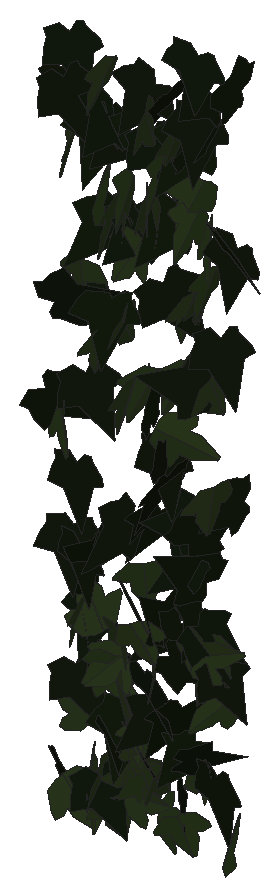
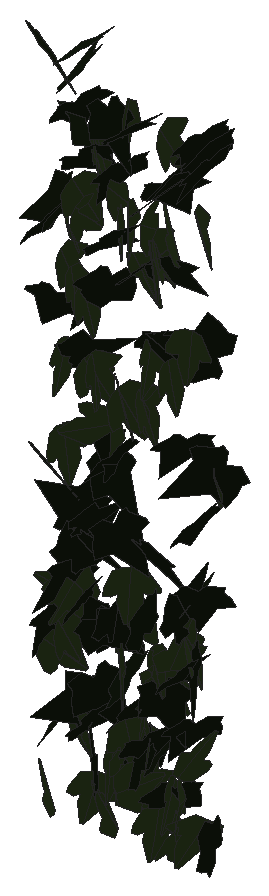
# SketchUp Ruby script. Lengths in inches.
U = 1.inch
M = Sketchup.active_model
def pt(a) = Geom::Point3d.new(a.map { |v| v * U })
def face(e, loops, mat)
  f = e.add_face(loops[0].map { |a| pt(a) })
  loops[1..].each { |l| e.add_face(l.map { |a| pt(a) }).erase! }
  f.material = f.back_material = mat if mat
  f
end
# faces: each face lists its corners as indices into pts; further lists are holes
def faces(e, pts, list, mat = nil) = list.each { |f| face(e, (f[0].is_a?(Array) ? f : [f]).map { |l| l.map { |i| pts[i] } }, mat) }
# xy, xz, yz: faces in a plane at the given z, y or x. An outline is a flat list of corners, or four numbers for a rectangle; further outlines are holes
def ring(l) = l.size == 4 ? [[l[0], l[1]], [l[2], l[1]], [l[2], l[3]], [l[0], l[3]]] : l.each_slice(2).to_a
def flat(e, list, mat, &to3) = list.each { |f| face(e, (f[0].is_a?(Array) ? f : [f]).map { |l| ring(l).map { |u, v| to3.(u, v) } }, mat) }
def xy(e, z, list, mat = nil) = flat(e, list, mat) { |x, y| [x, y, z] }
def xz(e, y, list, mat = nil) = flat(e, list, mat) { |x, z| [x, y, z] }
def yz(e, x, list, mat = nil) = flat(e, list, mat) { |y, z| [x, y, z] }
def lines(e, pts, list) = list.each { |a, b| e.add_line(pt(pts[a]), pt(pts[b])) }
# prism: a flat outline (further loops are holes) pulled along v
def prism(e, loops, v, mat = nil)
  f = face(e, loops, mat); d = Geom::Vector3d.new(v.map { |x| x * U })
  f.pushpull(f.normal.samedirection?(d) ? d.length : -d.length)
end
def box(e, o, s, mat = nil) = prism(e, [[o, [o[0] + s[0], o[1], o[2]], [o[0] + s[0], o[1] + s[1], o[2]], [o[0], o[1] + s[1], o[2]]]], [0, 0, s[2]], mat)
def at(x, y, z, deg = 0) = Geom::Transformation.translation(pt([x, y, z])) * Geom::Transformation.rotation(ORIGIN, Z_AXIS, deg.degrees)
def axes(o, x, y, z) = Geom::Transformation.new([*x, 0, *y, 0, *z, 0, *pt(o).to_a, 1])
def part(name) = M.definitions.add(name)
# library, detail: a bought-in or finely detailed component or shape, given as its bounding box
def library(name, o, s) = part(name).tap { |d| box(d.entities, o, s) }
def detail(e, o, s) = box(e.add_group.entities, o, s)
def put(e, d, t, mat = nil) = e.add_instance(d, t).tap { |i| i.material = mat if mat }
def group(e, t, mat = nil) = e.add_group.tap { |g| g.transformation = t; g.material = mat if mat }.entities
root = M.entities
M.materials.add("efeu1").color = [18, 25, 13]
M.materials.add("efeu2").color = [43, 57, 29]
c1 = part("ivyleaf_9")
p = [[1.54,2.16,1.25],[1.36,2.04,1.19],[-0.21,0.99,0.68],[-0.71,1.11,0.82],[-0.85,0.86,0.67],[-0.8,0.17,0.21],
  [-0.9,-0.01,0.1],[-0.67,-0.16,-0.02],[-0.08,-0.08,-0.05],[-0.03,-0.6,-0.4],[0.65,-0.88,-0.66],[0.83,-0.6,-0.49],
  [1.29,-0.42,-0.43],[1.8125,-0.07,-0.26],[1.21,0.44,0.15]]
faces(c1.entities,p,[[0,1,2,3,4,5,6,7,8,9,10,11,12,13,14]],"efeu1")
c2 = part("ivyleaf_10")
p = [[0,0.5,-0.03],[-0.0625,2.02,-0.43],[-0.19,2.01,-0.46],[-0.54,1.05,-0.29],[-0.52,0.625,-0.18],[-0.83,0.76,-0.28],
  [-1.16,0.64,-0.33],[-1.15,0.33,-0.24],[-0.77,-0.39,0.02],[-0.3,-0.51,0.16],[0.04,-0.48,0.23],[-0.02,2.01,-0.4375],
  [-0.06,2.01,-0.43],[0.04,-0.49,0.23],[0.67,-0.49,0.14],[1.38,0.36,-0.2],[1.375,0.51,-0.24],[0.81,0.65,-0.19],
  [0.62,0.59,-0.15],[0.6,1.09,-0.28],[0.5,1.23,-0.31]]
faces(c2.entities,p,[[0,1,2,3,4,5,6,7,8,9,10],[11,12,0,13,14,15,16,17,18,19,20]],"efeu2")
put(root,c1,axes([551.33,129.59,209.66],[0.30816,-0.97245,0.26451],[0.08754,-0.24973,-1.02008],[1.00398,0.32026,0.00775]))
put(root,c1,axes([543.79,129.1,239.86],[0.16795,-0.91073,-0.55695],[-0.07762,0.5519,-0.92587],[1.06471,0.1839,0.02036]))
put(root,c2,axes([548.23,128.8,239.77],[0.29173,-0.86162,-0.5234],[0.03321,0.55279,-0.89149],[1.00759,0.23125,0.18093]))
put(root,c2,axes([543.08,129.5,224.16],[0.54325,-0.33773,0.8446],[0.78802,-0.31665,-0.63348],[0.45435,0.953,0.08883]))
put(root,c1,axes([550.39,129.99,241.25],[-0.30308,-0.60694,0.7858],[0.06583,-0.83207,-0.61729],[0.99072,-0.13039,0.28141]))
put(root,c2,axes([551.37,129.22,223.13],[-0.21403,-1.02754,-0.02071],[0.00508,0.0201,-1.04959],[1.02773,-0.21409,0.00087]))
put(root,c2,axes([547.5625,129.05,215.5],[-0.80699,-0.17302,-0.36482],[0.36747,0.02312,-0.82382],[0.16731,-0.88532,0.04978]))
put(root,c1,axes([550.58,129.62,227.51],[-0.39565,0.02717,0.90439],[-0.85568,-0.33206,-0.36436],[0.29408,-0.92962,0.15658]))
put(root,c1,axes([543.59,128.86,229.57],[0.34005,0.02572,1.00838],[1.00834,-0.03717,-0.33909],[0.02701,1.06352,-0.03623]))
put(root,c2,axes([550.67,128.97,215.37],[-0.35587,-0.23953,1.03534],[0.9324,0.45346,0.42539],[-0.50984,0.99647,0.05529]))
put(root,c2,axes([546.91,129.43,226.48],[0.26737,-1.04337,0.12862],[0.03423,-0.124,-1.07708],[1.05071,0.26954,0.00236]))
put(root,c1,axes([545.54,129.15,207.95],[-0.06378,-0.73332,-0.67601],[0.05403,0.67386,-0.73608],[0.99591,-0.08352,-0.00335]))
put(root,c1,axes([544.09,129.77,217.86],[0.21966,-0.90955,0.34178],[0.13037,-0.31964,-0.93444],[0.96286,0.25078,0.04856]))
put(root,c2,axes([547.12,129.3,207.49],[-0.23624,0.00028,0.98914],[0.98473,0.09606,0.23516],[-0.09337,1.01242,-0.02259]))
put(root,c1,axes([543.95,129.68,221.7],[0.09609,-0.96582,-0.0051],[-0.00047,0.00507,-0.97059],[0.96583,0.09609,0.00003]))
put(root,c1,axes([550,129.9375,242.71],[-0.10891,-0.96056,0.28969],[0.27491,-0.30881,-0.9206],[0.96489,-0.02044,0.29499]))
put(root,c1,axes([545.72,129.87,209.85],[0.1744,-0.68198,0.53825],[0.17856,-0.50913,-0.70294],[0.85025,0.24681,0.03722]))
put(root,c2,axes([546.37,129.97,235.375],[0.09384,-0.52453,0.8809],[0.54111,-0.726,-0.48994],[0.87081,0.50765,0.20952]))
put(root,c1,axes([545.76,129.65,230.04],[-0.61638,-0.68009,-0.36267],[0.24583,0.26666,-0.91784],[0.73049,-0.66358,0.00286]))
put(root,c2,axes([544.3125,129.55,215.45],[0.4068,-0.87935,0.13467],[0.05007,-0.12521,-0.96886],[0.88819,0.40981,-0.00706]))
put(root,c1,axes([547.46,129.76,213.06],[0.53178,-0.87396,0.39802],[0.22613,-0.32822,-1.02282],[0.93333,0.57748,0.02103]))
put(root,c1,axes([548.86,129.41,222.89],[-0.43908,0.84469,-0.55493],[0.24873,-0.49611,-0.95197],[-0.97958,-0.50459,0.00702]))
put(root,c1,axes([549.37,129.11,214.9],[0.23619,-0.01945,-0.87995],[0.62428,0.64595,0.15329],[0.62045,-0.64253,0.18074]))
put(root,c2,axes([545.83,129.77,234.4],[0.45874,-0.91889,0.39791],[0.16359,-0.36302,-1.02693],[0.98789,0.48681,-0.01472]))
put(root,c2,axes([551.53,129.83,213.15],[-0.38198,-0.4071,0.73145],[-0.34621,-0.65519,-0.54546],[0.76216,-0.50165,0.11882]))
put(root,c2,axes([545.46,129.45,228.42],[-0.00779,-0.95669,-0.01264],[0.00015,0.01263,-0.95672],[0.95677,-0.00779,0.00004]))
put(root,c1,axes([547.65,130.09,211.07],[-0.28926,-0.58968,0.59581],[-0.2344,-0.54825,-0.65641],[0.80485,-0.3716,0.02297]))
put(root,c2,axes([545.11,129.65,234.41],[0.65992,-0.82122,-0.43743],[0.25988,-0.35225,1.05338],[-0.89342,-0.70905,-0.01669]))
put(root,c1,axes([550.27,129.84,239.99],[-0.21869,-0.97219,-0.06189],[0.00757,0.06173,-0.99647],[0.97413,-0.21873,-0.00615]))
put(root,c2,axes([547.15,129.41,233.1],[0.89274,-0.27797,-0.42476],[-0.39705,0.15304,-0.93466],[0.31628,0.97672,0.02557]))
put(root,c2,axes([544.61,129.96,208.05],[-0.17802,0.37149,-0.87717],[0.24033,-0.84597,-0.40705],[-0.92178,-0.29231,0.06327]))
put(root,c2,axes([546.79,129.64,208.18],[-0.57066,-0.66814,-0.14881],[-0.0784,-0.12867,0.87835],[-0.68,0.57553,0.02362]))
put(root,c1,axes([551.51,129.62,230.16],[-0.42266,-0.57459,-0.69219],[0.58154,0.40898,-0.69459],[0.68636,-0.70036,0.16227]))
put(root,c2,axes([547.83,129.25,208.64],[-0.43732,-0.78,-0.32184],[0.15923,0.27969,-0.89423],[0.82863,-0.46541,0.00198]))
put(root,c1,axes([550.28,128.84,210.48],[0.58085,0.27349,0.64911],[0.52623,0.39077,-0.63553],[-0.46821,0.77847,0.09098]))
put(root,c1,axes([549.38,129.64,212.2],[-0.02229,0.6239,-0.76266],[-0.03791,-0.76283,-0.62293],[-0.98461,0.01524,0.04125]))
put(root,c2,axes([548.4,129.3,235.1],[0.61291,-0.69917,-0.36837],[-0.10099,0.39306,-0.91405],[0.78379,0.59738,0.17029]))
put(root,c1,axes([545.61,129.95,233.72],[-0.87275,-0.40517,0.12381],[-0.1085,-0.06032,-0.96217],[0.40954,-0.87942,0.00895]))
put(root,c1,axes([550.9,129.06,216.81],[0.16706,-0.33779,-0.8306],[-0.09858,0.83285,-0.35853],[0.89122,0.15544,0.11604]))
put(root,c2,axes([546.09,129.58,213.45],[0.77037,-0.01339,-0.6543],[-0.65355,0.03664,-0.77025],[0.03392,1.01007,0.01927]))
put(root,c1,axes([546.37,130.17,215.87],[0.20956,-0.48225,0.93208],[0.41962,-0.83269,-0.52517],[0.9619,0.46832,0.02604]))
put(root,c2,axes([549.64,130.22,235.03],[-0.17617,-0.66482,0.74787],[0.28215,-0.76156,-0.61053],[0.96004,0.10183,0.31667]))
put(root,c2,axes([547.65,129.47,235.34],[0.40038,-0.85297,-0.25877],[0.04779,0.30381,-0.92749],[0.89007,0.36738,0.1662]))
put(root,c2,axes([550.67,129.42,209.91],[0.61794,-0.32297,-0.59003],[-0.46629,0.37176,-0.69185],[0.48478,0.76927,0.08663]))
put(root,c2,axes([547.97,130.19,236.65],[0.18269,-0.60037,0.75677],[0.38449,-0.66135,-0.61749],[0.88618,0.41072,0.1119]))
put(root,c2,axes([545.71,129.63,213.24],[-0.72731,-0.43098,0.27772],[-0.25377,-0.11622,-0.84495],[0.4455,-0.7698,-0.02792]))
put(root,c2,axes([546.67,129.29,212.35],[-0.48407,0.85664,0.25934],[-0.14284,0.21712,-0.9838],[-0.88356,-0.50442,0.01697]))
put(root,c2,axes([545.54,129.15,207.98],[0.10551,-0.67668,-0.72818],[-0.03621,0.72917,-0.68284],[0.99339,0.09845,0.05245]))
put(root,c2,axes([549.53,129.51,207.08],[-0.73134,-0.4943,-0.20702],[0.18107,0.10172,-0.88256],[0.50438,-0.75323,0.01667]))
put(root,c1,axes([549.06,130.07,207.48],[-0.02568,0.14488,0.90595],[0.17864,-0.88817,0.1471],[0.8999,0.18044,-0.00335]))
put(root,c2,axes([545.42,129.61,212.68],[-0.47952,-0.19549,-0.72079],[0.74557,-0.07556,-0.47551],[0.04338,-0.86242,0.20505]))
put(root,c1,axes([550.11,130.24,218.22],[0.0954,0.07332,1.01492],[-0.80361,-0.61989,0.12032],[0.62421,-0.80926,-0.00021]))
put(root,c1,axes([549.43,130.42,210.39],[-0.35826,-0.75572,0.52668],[-0.13698,-0.51512,-0.83231],[0.9109,-0.37469,0.08198]))
put(root,c1,axes([551.26,129.76,234.91],[0.76631,-0.5934,0.19678],[0.1584,-0.11684,-0.9692],[0.60478,0.7825,0.00451]))
put(root,c1,axes([546.42,129.97,219.74],[-1.0184,0.03309,-0.08224],[0.08212,-0.00522,-1.01894],[-0.0334,-1.02171,0.00254]))
put(root,c1,axes([545.09,130.2,237.99],[-0.57129,-0.85782,-0.06748],[0.03468,0.05797,-1.03064],[0.85977,-0.57233,-0.00326]))
put(root,c1,axes([545.08,130.49,238.06],[-0.25303,-0.72232,0.64363],[-0.02435,-0.66031,-0.75062],[0.96717,-0.2056,0.14949]))
put(root,c1,axes([546.49,130.24,209.18],[0.3244,-0.51928,0.8931],[0.468,-0.76067,-0.61227],[0.92101,0.56943,-0.00345]))
put(root,c1,axes([543.5625,129.93,218.55],[-0.49413,-0.69278,-0.4438],[0.24506,0.37026,-0.85083],[0.7854,-0.55139,-0.01374]))
put(root,c2,axes([550.97,129.59,215.96],[-0.86406,0.08888,-0.27068],[0.27113,-0.00894,-0.86843],[-0.0875,-0.90542,-0.018]))
put(root,c1,axes([546.61,130.55,233.31],[-0.47101,-0.65424,0.61164],[-0.02959,-0.67932,-0.74943],[0.89513,-0.36672,0.29706]))
put(root,c1,axes([548.75,129.45,231.86],[0.03596,-0.63583,-0.8599],[0.01876,0.86063,-0.63559],[1.06928,0.00628,0.04007]))
put(root,c2,axes([547.43,129.96,210.57],[-0.51462,-0.71785,0.2082],[0.04254,-0.28049,-0.86198],[0.74622,-0.47906,0.19272]))
put(root,c1,axes([551.42,129.625,214.83],[0.10118,-0.6731,-0.60781],[-0.11036,0.5979,-0.68049],[0.90017,0.14896,-0.0151]))
put(root,c1,axes([544.4,130.41,216.83],[0.09385,0.16673,1.04725],[-0.52122,-0.90834,0.19133],[0.92351,-0.5296,0.00155]))
put(root,c2,axes([546.03,129.65,206.68],[-0.55887,-0.73144,-0.18088],[0.10289,0.14901,-0.92047],[0.74642,-0.5682,-0.00855]))
put(root,c1,axes([552.53,129.54,242.25],[-0.72874,0.65171,0.28984],[-0.1953,0.21621,-0.97719],[-0.68599,-0.75387,-0.0297]))
put(root,c1,axes([546.1875,130.27,210.63],[-0.40529,-0.94033,-0.05742],[0.03289,0.04835,-1.0239],[0.94151,-0.40647,0.01105]))
put(root,c2,axes([543.8125,129.38,206.82],[0.45523,0.81473,0.53404],[0.24921,0.47246,-0.93322],[-0.94174,0.51885,0.0112]))
put(root,c2,axes([549.21,130.2,227.62],[-0.29568,-0.78757,0.49781],[-0.09027,-0.49561,-0.83769],[0.92732,-0.29936,0.07719]))
put(root,c1,axes([548.22,129.15,225.56],[-0.01969,0.20976,0.97191],[-0.23132,0.94446,-0.20852],[-0.967,-0.2302,0.03009]))
put(root,c2,axes([547.39,130.2,226.74],[-0.26306,-0.90601,0.45963],[-0.11023,-0.44653,-0.94328],[1.00993,-0.28473,0.01677]))
put(root,c2,axes([548.93,129.9375,238.77],[0.19827,-0.97173,0.0115],[0.00281,-0.01117,-0.99175],[0.9718,0.19829,0.00052]))
put(root,c1,axes([548.125,130.2,223.68],[0.11376,-1.01564,-0.05401],[-0.01226,0.05298,-1.02197],[1.017,0.11424,-0.00628]))
put(root,c1,axes([548.71,129.16,223.2],[-0.03557,-0.10437,0.99796],[0.27583,0.9591,0.11014],[-0.96475,0.27806,-0.0053]))
put(root,c2,axes([544.87,129.85,214.78],[0.28524,1.01027,0.21761],[-0.05785,-0.20978,1.04977],[1.03182,-0.29104,-0.0013]))
put(root,c2,axes([543.94,130.24,210.02],[-0.03503,0.77467,0.6225],[-0.03356,-0.62345,0.77397],[0.99322,0.00625,0.04811]))
put(root,c1,axes([549.82,130.11,219.17],[-0.89934,0.02943,0.11968],[-0.12014,-0.01275,-0.89967],[-0.02749,-0.90718,0.01653]))
put(root,c2,axes([544.98,130.33,240.31],[0.18872,-0.88894,0.47616],[0.09964,-0.46562,-0.90875],[1.0035,0.21341,0.00069]))
put(root,c1,axes([548.15,130.3125,215.33],[-0.01052,0.32907,0.84182],[-0.52981,-0.68432,0.26089],[0.73229,-0.49038,0.20084]))
put(root,c1,axes([551.58,130.5,234.02],[-0.06082,-0.94583,0.25251],[0.02365,-0.25434,-0.947],[0.97867,-0.05263,0.03857]))
put(root,c1,axes([548.27,130.63,234.28],[-0.5242,-0.72669,0.37742],[-0.0703,-0.40653,-0.8804],[0.81583,-0.50196,0.16664]))
put(root,c2,axes([547.36,129.87,217.89],[-0.72559,-0.62656,-0.03145],[0.0232,0.02126,-0.95867],[0.62692,-0.72596,-0.00093]))
put(root,c2,axes([546.08,130.27,210.84],[-0.38166,0.43036,-0.66955],[0.288,-0.61757,-0.56112],[-0.742,-0.46107,0.12661]))
put(root,c1,axes([550.29,129.15,238.52],[0.28428,0.53541,0.79457],[-0.27669,0.83937,-0.4666],[-0.9173,-0.08725,0.38698]))
put(root,c2,axes([548.69,129.74,224.83],[-0.40521,-0.10733,-1.03525],[1.03488,0.07673,-0.41303],[0.11081,-1.10908,0.07161]))
put(root,c1,axes([543.74,129.95,212.12],[0.00984,-0.78855,-0.55731],[0.15303,0.55157,-0.77772],[0.95341,-0.08039,0.13059]))
put(root,c2,axes([549.75,130.375,236.23],[-0.39343,-0.74862,0.505],[-0.02046,-0.54332,-0.82136],[0.90279,-0.33855,0.20146]))
put(root,c2,axes([547.09,130.49,208.07],[-0.22743,0.00124,-0.85488],[-0.577,-0.65295,0.15256],[-0.63079,0.59682,0.16868]))
put(root,c1,axes([543.03,129.93,239.68],[0.39747,-0.85339,-0.43074],[-0.08238,0.43417,-0.93621],[0.95238,0.39372,0.09878]))
put(root,c2,axes([550.52,130.35,214.55],[0.05641,-0.83868,0.42223],[0.10548,-0.41465,-0.83772],[0.93302,0.09758,0.06918]))
put(root,c2,axes([550.47,130.29,232.53],[0.1134,-0.91043,0.32112],[0.08376,-0.31283,-0.91651],[0.96176,0.13459,0.04196]))
put(root,c1,axes([548.65,130.375,215.59],[0.0484,0.1256,-0.88774],[-0.21365,-0.86181,-0.13358],[-0.87075,0.21844,-0.01657]))
put(root,c2,axes([550.18,130.43,234.4],[0.55277,-0.35932,0.77542],[0.63703,-0.44238,-0.65911],[0.56972,0.84328,-0.01536]))
put(root,c2,axes([549.49,130.13,231.06],[0.02764,-0.96666,0.06985],[0.0297,-0.069,-0.96666],[0.96873,0.0297,0.02764]))
put(root,c1,axes([547.0625,130.77,240.02],[-0.48746,-0.78571,0.4364],[0.03228,-0.51144,-0.88475],[0.89818,-0.40803,0.26864]))
put(root,c2,axes([549.14,129.93,227.68],[0.12716,-0.92573,-0.21991],[0.01949,0.22436,-0.93316],[0.95129,0.11914,0.04851]))
put(root,c2,axes([550.88,129.76,227.78],[-0.03911,-0.88003,-0.43626],[0.14265,0.42688,-0.87391],[0.97181,-0.09807,0.11072]))
put(root,c1,axes([542.62,129.46,224.85],[0.06027,0.00922,-1.05526],[0.31753,1.00784,0.02694],[1.0064,-0.31854,0.05469]))
put(root,c1,axes([549.6,130.7,216.2],[-0.07164,-0.73855,0.50918],[-0.05478,-0.50624,-0.742],[0.89538,-0.09006,-0.00466]))
put(root,c2,axes([546.12,129.64,214.4],[0.56241,-0.15638,-0.72137],[-0.45072,0.64544,-0.49131],[0.58454,0.64814,0.31522]))
put(root,c1,axes([544.15,130.0625,225.78],[-0.05174,-0.77447,-0.6047],[0.20348,0.58397,-0.76533],[0.96129,-0.1653,0.12946]))
put(root,c2,axes([543.26,130.2,236.74],[0.57165,-0.87708,0.00525],[-0.00003,-0.00628,-1.04692],[0.87709,0.57164,-0.00345]))
put(root,c2,axes([547.96,130.42,206.25],[0.31515,-0.26489,-0.90917],[0.7002,-0.57992,0.41167],[-0.63755,-0.76785,0.00272]))
put(root,c2,axes([547.96,129.6875,213.85],[0.48655,-0.71146,-0.68703],[-0.24723,0.65386,-0.85221],[0.95763,0.53028,0.12904]))
put(root,c1,axes([547.76,130.29,220.53],[0.0486,0.54046,-0.76429],[-0.03053,-0.764,-0.54219],[-0.93558,0.05301,-0.02201]))
put(root,c2,axes([546.11,129.85,234.125],[0.60903,-0.59378,-0.46952],[-0.19661,0.45785,-0.83406],[0.73101,0.61785,0.16685]))
put(root,c2,axes([548.32,129.72,208.95],[0.09669,-0.83212,-0.61124],[-0.05469,0.60893,-0.83762],[1.03105,0.11034,0.01289]))
put(root,c2,axes([546.31,129.72,229.19],[0.04118,-0.79093,-0.60404],[-0.02471,0.60356,-0.79199],[0.9949,0.04773,0.00533]))
put(root,c1,axes([549.86,129.7,220.18],[-0.06031,-0.10418,0.94422],[0.90925,0.26763,0.08761],[-0.27507,0.9075,0.08256]))
put(root,c1,axes([542.33,130.47,206.84],[0.52768,-0.13411,-0.73594],[0.7375,-0.0575,0.53928],[-0.12523,-0.90374,0.07489]))
put(root,c1,axes([547.5,130.17,238.01],[0.15958,-0.87496,-0.4627],[0.02422,0.47199,-0.88417],[0.98948,0.12956,0.09627]))
put(root,c2,axes([548.99,129.99,238.8],[0.33802,-0.86532,-0.34696],[-0.06972,0.34457,-0.92727],[0.92968,0.34046,0.05661]))
put(root,c1,axes([543.98,129.74,215.39],[0.37913,-0.0199,-0.91772],[-0.90583,0.15265,-0.37752],[0.14862,0.98115,0.04012]))
put(root,c1,axes([545.38,130.07,213.27],[0.29322,0.45519,-0.70167],[-0.49884,-0.50164,-0.53389],[-0.67134,0.57155,0.09024]))
put(root,c1,axes([548.38,130.03,240.34],[-0.33718,0.88364,-0.32096],[0.11984,-0.29779,-0.94577],[-0.93245,-0.3578,-0.00549]))
put(root,c1,axes([545.49,130.98,237.22],[-0.44199,-0.66489,0.62532],[-0.01331,-0.69,-0.74308],[0.91265,-0.33206,0.292]))
put(root,c2,axes([551.4375,130.1875,205.83],[0.65096,-0.73981,-0.07337],[0.04907,-0.05456,0.98543],[-0.74182,-0.6528,0.00079]))
put(root,c1,axes([552.09,130.22,222.59],[-0.84648,0.36065,0.05804],[-0.05481,0.01943,-0.9201],[-0.36116,-0.84825,0.0036]))
put(root,c1,axes([544.1,130.81,214.73],[-0.20876,-0.86829,0.31305],[0.02592,-0.32634,-0.88788],[0.92264,-0.18729,0.09578]))
put(root,c2,axes([544.59,130.29,206.54],[0.04314,0.82699,-0.28665],[-0.03558,-0.2851,-0.82788],[-0.87453,0.0524,0.01954]))
put(root,c1,axes([549.29,130.81,220.22],[-0.4066,-0.07875,0.80711],[-0.56719,-0.61768,-0.346],[0.57959,-0.65971,0.22761]))
put(root,c2,axes([550.12,130.19,231.66],[0.18455,-0.94079,-0.16334],[-0.03338,0.15991,-0.95872],[0.95428,0.18753,-0.00194]))
put(root,c1,axes([549.2,130.85,238.22],[-0.65644,-0.74587,0.19918],[-0.06287,-0.20893,-0.98959],[0.76944,-0.6534,0.08907]))
put(root,c2,axes([543.93,130.15,230.71],[-0.95406,0.0196,0.0646],[-0.06623,-0.09508,-0.9494],[-0.01304,-0.9515,0.0962]))
put(root,c1,axes([543.05,130.38,241.125],[0.13356,-0.94746,-0.32727],[0.04035,0.33498,-0.95331],[1.00158,0.11285,0.08204]))
